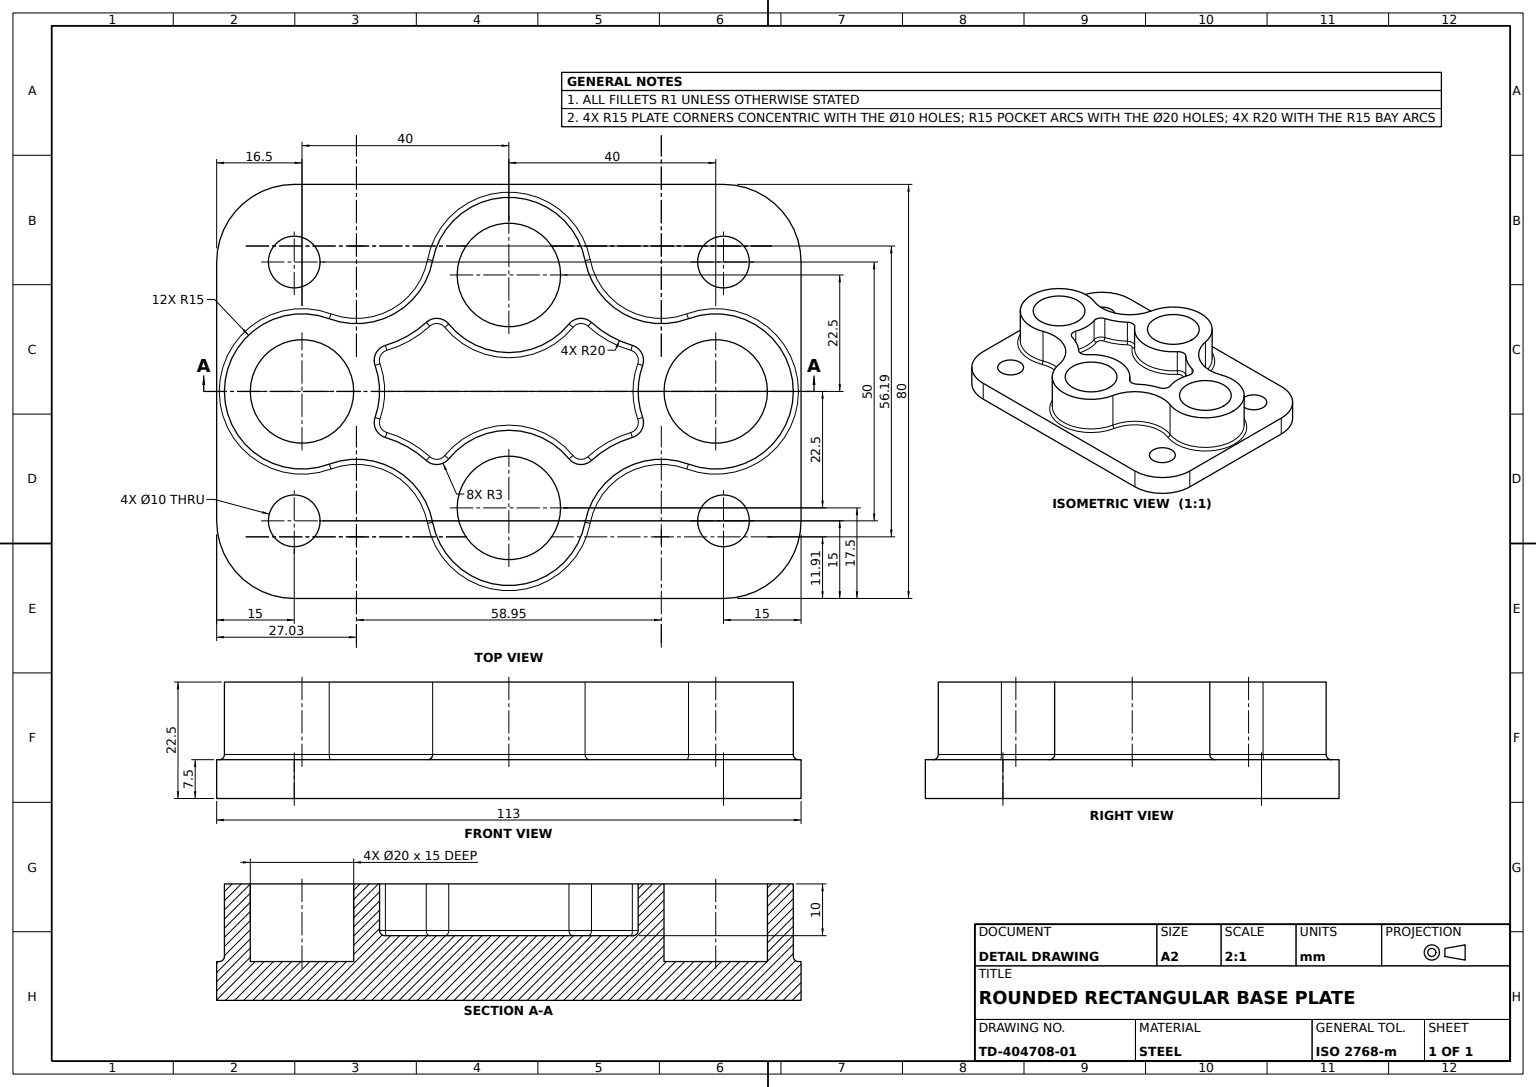
solid
v1 (0,22.5,-30)
v2 (0,7.5,-30)
e1 v1 v2 LINE
v3 (0,7.5,-50)
e2 v2 v3 CIRCLE(AX(P(0,7.5,-40),D(0,-1,0),D(0,0,1)),10)
v4 (0,22.5,-50)
e3 v4 v3 LINE
e4 v4 v1 CIRCLE(AX(P(0,22.5,-40),D(0,1,0),D(0,0,1)),10)
face CYL(AX(P(0,22.5,-40),D(0,-1,0),D(0,0,-1)),10) rev [e1 e2 -e3 e4]
v5 (5.01068,13.5,-25.861645)
v6 (8.892813,13.5,-23.873986)
e5 v5 v6 CIRCLE(AX(P(6.012816,13.5,-23.033974),D(0,-1,0),D(0,0,1)),3)
v7 (8.892813,22.5,-23.873986)
e6 v6 v7 LINE
v8 (5.01068,22.5,-25.861645)
e7 v7 v8 CIRCLE(AX(P(6.012816,22.5,-23.033974),D(0,1,0),D(0,0,-1)),3)
e8 v5 v8 LINE
face CYL(AX(P(6.012816,12.5,-23.033974),D(0,1,0),D(0,0,1)),3) rev [e5 e6 e7 -e8]
v9 (12.598841,12.5,-15.298823)
v10 (7.932814,12.5,-23.593982)
e9 v9 v10 CIRCLE(AX(P(28.092789,12.5,-29.474069),D(0,-1,0),D(0,0,1)),21)
v11 (13.336648,13.5,-15.973835)
e10 v9 v11 CIRCLE(AX(P(12.598841,13.5,-15.298823),D(0.675011674,0,0.737807048),D(0.737807048,0,-0.675011674)),1)
e11 v6 v11 CIRCLE(AX(P(28.092789,13.5,-29.474069),D(0,1,0),D(0,0,1)),20)
e12 v10 v6 CIRCLE(AX(P(7.932814,13.5,-23.593982),D(0.280004116,0,0.9599988),D(0.9599988,0,-0.280004116)),1)
face TORUS(AX(P(28.092789,13.5,-29.474069),D(0,1,0),D(0,0,1)),21,1) rev [-e9 e10 -e11 -e12]
v12 (0,7.5,50)
v13 (0,7.5,30)
e13 v12 v13 CIRCLE(AX(P(0,7.5,40),D(0,-1,0),D(0,0,1)),10)
e14 v13 v12 CIRCLE(AX(P(0,7.5,40),D(0,-1,0),D(0,0,1)),10)
face PLANE(AX(P(-25,7.5,41.5),D(0,1,0),D(0,0,1))) [-e13 -e14]
v14 (-8.892813,13.5,-23.873986)
v15 (-8.892813,22.5,-23.873986)
e15 v14 v15 LINE
v16 (-13.336648,22.5,-15.973835)
e16 v15 v16 CIRCLE(AX(P(-28.092789,22.5,-29.474069),D(0,-1,0),D(0,0,-1)),20)
v17 (-13.336648,13.5,-15.973835)
e17 v17 v16 LINE
e18 v17 v14 CIRCLE(AX(P(-28.092789,13.5,-29.474069),D(0,1,0),D(0,0,1)),20)
face CYL(AX(P(-28.092789,12.5,-29.474069),D(0,1,0),D(0,0,1)),20) [e15 e16 -e17 e18]
e19 v3 v2 CIRCLE(AX(P(0,7.5,-40),D(0,-1,0),D(0,0,1)),10)
face PLANE(AX(P(-25,7.5,41.5),D(0,1,0),D(0,0,1))) [-e2 -e19]
v18 (0,22.5,30)
e20 v18 v13 LINE
v19 (0,22.5,50)
e21 v18 v19 CIRCLE(AX(P(0,22.5,40),D(0,1,0),D(0,0,1)),10)
e22 v19 v12 LINE
face CYL(AX(P(0,22.5,40),D(0,-1,0),D(0,0,-1)),10) rev [-e20 e21 e22 e13]
v20 (-6.012816,12.5,25.033974)
v21 (-6.012816,13.5,26.033974)
e23 v20 v21 CIRCLE(AX(P(-6.012816,13.5,25.033974),D(-1,0,0),D(0,0,1)),1)
v22 (-5.01068,13.5,25.861645)
e24 v22 v21 CIRCLE(AX(P(-6.012816,13.5,23.033974),D(0,-1,0),D(0,0,1)),3)
v23 (-5.344724,12.5,24.919087)
e25 v22 v23 CIRCLE(AX(P(-5.344724,13.5,24.919087),D(0.942557427,0,-0.334044155),D(-0.334044155,0,-0.942557427)),1)
e26 v20 v23 CIRCLE(AX(P(-6.012816,12.5,23.033974),D(0,1,0),D(0,0,1)),2)
face TORUS(AX(P(-6.012816,13.5,23.033974),D(0,1,0),D(0,0,1)),2,1) rev [e23 -e24 e25 -e26]
v24 (5.01068,13.5,25.861645)
v25 (5.344724,12.5,24.919087)
e27 v24 v25 CIRCLE(AX(P(5.344724,13.5,24.919087),D(0.942557427,0,0.334044155),D(0.334044155,0,-0.942557427)),1)
v26 (6.012814,13.5,26.033973)
e28 v26 v24 CIRCLE(AX(P(6.012814,13.5,23.033969),D(0,-1,0),D(0,0,1)),3.000004)
v27 (6.012814,12.5,25.033973)
e29 v27 v26 CIRCLE(AX(P(6.012814,13.5,25.033973),D(-1,0,0),D(0,0,1)),1)
e30 v25 v27 CIRCLE(AX(P(6.012814,12.5,23.033969),D(0,1,0),D(0,0,1)),2.000004)
face TORUS(AX(P(6.012814,13.5,23.033969),D(0,1,0),D(0,0,1)),2.000004,1) rev [-e27 -e28 -e29 -e30]
v28 (25.296394,8.5,-14.737034)
v29 (14.046394,8.5,-34.737034)
e31 v28 v29 CIRCLE(AX(P(28.092789,8.5,-29.474069),D(0,-1,0),D(0,0,1)),15)
v30 (25.482821,7.5,-15.719503)
e32 v30 v28 CIRCLE(AX(P(25.482821,8.5,-15.719503),D(-0.982468951,0,-0.186426284),D(-0.186426284,0,0.982468951)),1)
v31 (14.982821,7.5,-34.38617)
e33 v31 v30 CIRCLE(AX(P(28.092789,7.5,-29.474069),D(0,1,0),D(0,0,1)),14)
e34 v31 v29 CIRCLE(AX(P(14.982821,8.5,-34.38617),D(0.350864382,0,-0.936426284),D(-0.936426284,0,-0.350864382)),1)
face TORUS(AX(P(28.092789,8.5,-29.474069),D(0,1,0),D(0,0,1)),14,1) rev [-e31 -e32 -e33 e34]
v32 (25,0,-36.5)
v33 (25,0,-46.5)
e35 v32 v33 CIRCLE(AX(P(25,0,-41.5),D(0,1,0),D(0,0,1)),5)
v34 (25,7.5,-36.5)
e36 v34 v32 LINE
v35 (25,7.5,-46.5)
e37 v34 v35 CIRCLE(AX(P(25,7.5,-41.5),D(0,1,0),D(0,0,1)),5)
e38 v35 v33 LINE
face CYL(AX(P(25,7.5,-41.5),D(0,-1,0),D(0,0,-1)),5) rev [-e35 -e36 e37 e38]
v36 (25,7.5,46.5)
v37 (25,0,46.5)
e39 v36 v37 LINE
v38 (25,7.5,36.5)
e40 v36 v38 CIRCLE(AX(P(25,7.5,41.5),D(0,1,0),D(0,0,1)),5)
v39 (25,0,36.5)
e41 v38 v39 LINE
e42 v37 v39 CIRCLE(AX(P(25,0,41.5),D(0,1,0),D(0,0,1)),5)
face CYL(AX(P(25,7.5,41.5),D(0,-1,0),D(0,0,-1)),5) rev [-e39 e40 e41 -e42]
v40 (-14.046394,8.5,34.737034)
v41 (0,8.5,55)
e43 v40 v41 CIRCLE(AX(P(0,8.5,40),D(0,1,0),D(0,0,1)),15)
v42 (-14.982821,7.5,34.38617)
e44 v40 v42 CIRCLE(AX(P(-14.982821,8.5,34.38617),D(0.350864382,0,-0.936426284),D(-0.936426284,0,-0.350864382)),1)
v43 (0,7.5,56)
e45 v43 v42 CIRCLE(AX(P(0,7.5,40),D(0,-1,0),D(0,0,1)),16)
e46 v41 v43 CIRCLE(AX(P(0,8.5,56),D(-1,0,0),D(0,0,1)),1)
face TORUS(AX(P(0,8.5,40),D(0,1,0),D(0,0,1)),16,1) rev [-e43 e44 -e45 -e46]
v44 (13.336648,13.5,15.973835)
v45 (13.336648,22.5,15.973835)
e47 v44 v45 LINE
v46 (8.892813,13.5,23.873986)
e48 v44 v46 CIRCLE(AX(P(28.092885,13.5,29.474123),D(0,1,0),D(0,0,1)),20.000108)
v47 (8.892813,22.5,23.873986)
e49 v46 v47 LINE
e50 v47 v45 CIRCLE(AX(P(28.092885,22.5,29.474123),D(0,-1,0),D(0,0,-1)),20.000108)
face CYL(AX(P(28.092885,12.5,29.474123),D(0,1,0),D(0,0,1)),20.000108) [-e47 e48 e49 e50]
v48 (22.5,7.5,-10)
v49 (22.5,7.5,10)
e51 v48 v49 CIRCLE(AX(P(22.5,7.5,0),D(0,-1,0),D(0,0,1)),10)
e52 v49 v48 CIRCLE(AX(P(22.5,7.5,0),D(0,-1,0),D(0,0,1)),10)
face PLANE(AX(P(-25,7.5,41.5),D(0,1,0),D(0,0,1))) [-e51 -e52]
v50 (-25.296394,22.5,-14.737034)
v51 (-25.296394,8.5,-14.737034)
e53 v50 v51 LINE
v52 (-25.296394,8.5,14.737034)
e54 v51 v52 CIRCLE(AX(P(-22.5,8.5,0),D(0,1,0),D(0,0,1)),15)
v53 (-25.296394,22.5,14.737034)
e55 v53 v52 LINE
e56 v50 v53 CIRCLE(AX(P(-22.5,22.5,0),D(0,1,0),D(0,0,1)),15)
face CYL(AX(P(-22.5,22.5,0),D(0,-1,0),D(0,0,-1)),15) [e53 e54 -e55 -e56]
e57 v39 v37 CIRCLE(AX(P(25,0,41.5),D(0,1,0),D(0,0,1)),5)
e58 v38 v36 CIRCLE(AX(P(25,7.5,41.5),D(0,1,0),D(0,0,1)),5)
face CYL(AX(P(25,7.5,41.5),D(0,-1,0),D(0,0,-1)),5) rev [e39 -e57 -e41 e58]
v54 (12.598841,12.5,15.298823)
e59 v44 v54 CIRCLE(AX(P(12.598841,13.5,15.298823),D(0.675011674,0,-0.737807048),D(-0.737807048,0,-0.675011674)),1)
v55 (7.932814,12.5,23.593981)
e60 v55 v54 CIRCLE(AX(P(28.092885,12.5,29.474123),D(0,-1,0),D(0,0,1)),21.000108)
e61 v46 v55 CIRCLE(AX(P(7.932814,13.5,23.593981),D(0.280005323,0,-0.959998447),D(-0.959998447,0,-0.280005323)),1)
face TORUS(AX(P(28.092885,13.5,29.474123),D(0,1,0),D(0,0,1)),21.000108,1) rev [-e48 e59 -e60 -e61]
v56 (-5.344725,12.5,-24.919088)
v57 (-7.932814,12.5,-23.593982)
e62 v56 v57 CIRCLE(AX(P(-6.012816,12.5,-23.033974),D(0,1,0),D(0,0,1)),2)
v58 (-5.01068,13.5,-25.861645)
e63 v56 v58 CIRCLE(AX(P(-5.344725,13.5,-24.919088),D(0.942557006,0,0.334045341),D(0.334045341,0,-0.942557006)),1)
e64 v14 v58 CIRCLE(AX(P(-6.012816,13.5,-23.033974),D(0,-1,0),D(0,0,1)),3)
e65 v57 v14 CIRCLE(AX(P(-7.932814,13.5,-23.593982),D(0.280004116,0,-0.9599988),D(-0.9599988,0,-0.280004116)),1)
face TORUS(AX(P(-6.012816,13.5,-23.033974),D(0,1,0),D(0,0,1)),2,1) rev [-e62 e63 -e64 -e65]
v59 (25,7.5,-56.5)
v60 (25,0,-56.5)
e66 v59 v60 LINE
v61 (-25,0,-56.5)
e67 v60 v61 LINE
v62 (-25,7.5,-56.5)
e68 v62 v61 LINE
e69 v59 v62 LINE
face PLANE(AX(P(-25,7.5,-56.5),D(0,0,1),D(1,0,0))) rev [e66 e67 -e68 -e69]
v63 (-12.598841,12.5,-15.298823)
e70 v63 v17 CIRCLE(AX(P(-12.598841,13.5,-15.298823),D(0.675011674,0,-0.737807048),D(-0.737807048,0,-0.675011674)),1)
e71 v57 v63 CIRCLE(AX(P(-28.092789,12.5,-29.474069),D(0,-1,0),D(0,0,1)),21)
face TORUS(AX(P(-28.092789,13.5,-29.474069),D(0,1,0),D(0,0,1)),21,1) rev [e65 -e18 -e70 -e71]
v64 (-13.019355,22.5,-11.624)
e72 v16 v64 CIRCLE(AX(P(-11.123226,22.5,-13.9488),D(0,1,0),D(0,0,1)),3)
v65 (-13.019355,13.5,-11.624)
e73 v65 v64 LINE
e74 v65 v17 CIRCLE(AX(P(-11.123226,13.5,-13.9488),D(0,-1,0),D(0,0,1)),3)
face CYL(AX(P(-11.123226,12.5,-13.9488),D(0,1,0),D(0,0,1)),3) rev [e17 e72 -e73 e74]
v66 (13.019355,22.5,11.624)
e75 v45 v66 CIRCLE(AX(P(11.123226,22.5,13.9488),D(0,1,0),D(0,0,1)),3)
v67 (13.019355,13.5,11.624)
e76 v67 v66 LINE
e77 v67 v44 CIRCLE(AX(P(11.123226,13.5,13.9488),D(0,-1,0),D(0,0,1)),3)
face CYL(AX(P(11.123226,12.5,13.9488),D(0,1,0),D(0,0,1)),3) rev [e47 e75 -e76 e77]
v68 (0,13.5,-25)
e78 v68 v5 CIRCLE(AX(P(0,13.5,-40),D(0,1,0),D(0,0,1)),15)
v69 (0,12.5,-24)
e79 v68 v69 CIRCLE(AX(P(0,13.5,-24),D(-1,0,0),D(0,0,1)),1)
v70 (5.344725,12.5,-24.919088)
e80 v70 v69 CIRCLE(AX(P(0,12.5,-40),D(0,-1,0),D(0,0,1)),16)
e81 v70 v5 CIRCLE(AX(P(5.344725,13.5,-24.919088),D(0.942557006,0,-0.334045341),D(-0.334045341,0,-0.942557006)),1)
face TORUS(AX(P(0,13.5,-40),D(0,1,0),D(0,0,1)),16,1) rev [-e78 e79 -e80 e81]
v71 (0,22.5,-25)
e82 v68 v71 LINE
v72 (-5.01068,22.5,-25.861645)
e83 v71 v72 CIRCLE(AX(P(0,22.5,-40),D(0,-1,0),D(0,0,1)),15)
e84 v58 v72 LINE
e85 v58 v68 CIRCLE(AX(P(0,13.5,-40),D(0,1,0),D(0,0,1)),15)
face CYL(AX(P(0,12.5,-40),D(0,1,0),D(0,0,1)),15) [e82 e83 -e84 e85]
e86 v33 v32 CIRCLE(AX(P(25,0,-41.5),D(0,1,0),D(0,0,1)),5)
v73 (-25,0,36.5)
v74 (-25,0,46.5)
e87 v73 v74 CIRCLE(AX(P(-25,0,41.5),D(0,1,0),D(0,0,1)),5)
e88 v74 v73 CIRCLE(AX(P(-25,0,41.5),D(0,1,0),D(0,0,1)),5)
v75 (-25,0,-46.5)
v76 (-25,0,-36.5)
e89 v75 v76 CIRCLE(AX(P(-25,0,-41.5),D(0,1,0),D(0,0,1)),5)
e90 v76 v75 CIRCLE(AX(P(-25,0,-41.5),D(0,1,0),D(0,0,1)),5)
v77 (-40,0,41.5)
v78 (-25,0,56.5)
e91 v77 v78 CIRCLE(AX(P(-25,0,41.5),D(0,1,0),D(0,0,1)),15)
v79 (-40,0,-41.5)
e92 v79 v77 LINE
e93 v61 v79 CIRCLE(AX(P(-25,0,-41.5),D(0,1,0),D(0,0,1)),15)
v80 (40,0,-41.5)
e94 v80 v60 CIRCLE(AX(P(25,0,-41.5),D(0,1,0),D(0,0,-1)),15)
v81 (40,0,41.5)
e95 v81 v80 LINE
v82 (25,0,56.5)
e96 v82 v81 CIRCLE(AX(P(25,0,41.5),D(0,1,0),D(0,0,1)),15)
e97 v78 v82 LINE
face PLANE(AX(P(-25,0,41.5),D(0,1,0),D(0,0,1))) rev [e42 e57] [e86 e35] [e87 e88] [e89 e90] [-e91 -e92 -e93 -e67 -e94 -e95 -e96 -e97]
v83 (22.5,22.5,-10)
e98 v83 v48 LINE
v84 (22.5,22.5,10)
e99 v83 v84 CIRCLE(AX(P(22.5,22.5,0),D(0,1,0),D(0,0,1)),10)
e100 v84 v49 LINE
face CYL(AX(P(22.5,22.5,0),D(0,-1,0),D(0,0,-1)),10) rev [e52 -e98 e99 e100]
e101 v24 v22 CIRCLE(AX(P(0,13.5,40.000056),D(0,1,0),D(0,0,1)),15.000053)
e102 v23 v25 CIRCLE(AX(P(0,12.5,40.000056),D(0,-1,0),D(0,0,1)),16.000053)
face TORUS(AX(P(0,13.5,40.000056),D(0,1,0),D(0,0,1)),16.000053,1) rev [-e101 e27 -e102 -e25]
v85 (-13.019355,22.5,11.624)
e103 v64 v85 CIRCLE(AX(P(-22.5,22.5,0),D(0,-1,0),D(0,0,-1)),15)
v86 (-13.019355,13.5,11.624)
e104 v86 v85 LINE
e105 v86 v65 CIRCLE(AX(P(-22.5,13.5,0),D(0,1,0),D(0,0,1)),15)
face CYL(AX(P(-22.5,12.5,0),D(0,1,0),D(0,0,1)),15) [e103 -e104 e105 e73]
v87 (-25.482821,7.5,-15.719503)
v88 (-14.982821,7.5,-34.38617)
e106 v87 v88 CIRCLE(AX(P(-28.092789,7.5,-29.474069),D(0,1,0),D(0,0,1)),14)
e107 v88 v31 CIRCLE(AX(P(0,7.5,-40),D(0,-1,0),D(0,0,1)),16)
v89 (25.482821,7.5,15.719503)
e108 v30 v89 CIRCLE(AX(P(22.5,7.5,0),D(0,-1,0),D(0,0,1)),16)
v90 (14.982821,7.5,34.38617)
e109 v89 v90 CIRCLE(AX(P(28.092789,7.5,29.474069),D(0,1,0),D(0,0,1)),14)
e110 v90 v43 CIRCLE(AX(P(0,7.5,40),D(0,-1,0),D(0,0,1)),16)
v91 (-25.482821,7.5,15.719503)
e111 v42 v91 CIRCLE(AX(P(-28.092789,7.5,29.474069),D(0,1,0),D(0,0,1)),14)
e112 v91 v87 CIRCLE(AX(P(-22.5,7.5,0),D(0,-1,0),D(0,0,1)),16)
e113 v35 v34 CIRCLE(AX(P(25,7.5,-41.5),D(0,1,0),D(0,0,1)),5)
v92 (-40,7.5,41.5)
v93 (-25,7.5,56.5)
e114 v92 v93 CIRCLE(AX(P(-25,7.5,41.5),D(0,1,0),D(0,0,1)),15)
v94 (25,7.5,56.5)
e115 v93 v94 LINE
v95 (40,7.5,41.5)
e116 v94 v95 CIRCLE(AX(P(25,7.5,41.5),D(0,1,0),D(0,0,1)),15)
v96 (40,7.5,-41.5)
e117 v95 v96 LINE
e118 v96 v59 CIRCLE(AX(P(25,7.5,-41.5),D(0,1,0),D(0,0,-1)),15)
v97 (-40,7.5,-41.5)
e119 v62 v97 CIRCLE(AX(P(-25,7.5,-41.5),D(0,1,0),D(0,0,1)),15)
e120 v97 v92 LINE
v98 (-25,7.5,36.5)
v99 (-25,7.5,46.5)
e121 v98 v99 CIRCLE(AX(P(-25,7.5,41.5),D(0,1,0),D(0,0,1)),5)
e122 v99 v98 CIRCLE(AX(P(-25,7.5,41.5),D(0,1,0),D(0,0,1)),5)
v100 (-25,7.5,-36.5)
v101 (-25,7.5,-46.5)
e123 v100 v101 CIRCLE(AX(P(-25,7.5,-41.5),D(0,1,0),D(0,0,1)),5)
e124 v101 v100 CIRCLE(AX(P(-25,7.5,-41.5),D(0,1,0),D(0,0,1)),5)
face PLANE(AX(P(-25,7.5,41.5),D(0,1,0),D(0,0,1))) [e106 e107 e33 e108 e109 e110 e45 e111 e112] [-e37 -e113] [e114 e115 e116 e117 e118 e69 e119 e120] [-e121 -e122] [-e123 -e124] [-e58 -e40]
e125 v72 v15 CIRCLE(AX(P(-6.012816,22.5,-23.033974),D(0,1,0),D(0,0,1)),3)
face CYL(AX(P(-6.012816,12.5,-23.033974),D(0,1,0),D(0,0,1)),3) rev [-e15 e64 e84 e125]
v102 (-12.387312,12.5,12.398933)
v103 (-12.598841,12.5,15.298823)
e126 v102 v103 CIRCLE(AX(P(-11.123226,12.5,13.9488),D(0,1,0),D(0,0,1)),2)
v104 (-7.932814,12.5,23.593982)
e127 v103 v104 CIRCLE(AX(P(-28.092789,12.5,29.474069),D(0,-1,0),D(0,0,1)),21)
e128 v104 v20 CIRCLE(AX(P(-6.012816,12.5,23.033974),D(0,1,0),D(0,0,1)),2)
e129 v27 v55 CIRCLE(AX(P(6.012814,12.5,23.033969),D(0,1,0),D(0,0,1)),2.000004)
v105 (12.387312,12.5,12.398933)
e130 v54 v105 CIRCLE(AX(P(11.123226,12.5,13.9488),D(0,1,0),D(0,0,1)),2)
v106 (12.387312,12.5,-12.398933)
e131 v105 v106 CIRCLE(AX(P(22.5,12.5,0),D(0,-1,0),D(0,0,1)),16)
e132 v106 v9 CIRCLE(AX(P(11.123226,12.5,-13.9488),D(0,1,0),D(0,0,1)),2)
e133 v10 v70 CIRCLE(AX(P(6.012816,12.5,-23.033974),D(0,1,0),D(0,0,1)),2)
e134 v69 v56 CIRCLE(AX(P(0,12.5,-40),D(0,-1,0),D(0,0,1)),16)
v107 (-12.387312,12.5,-12.398933)
e135 v63 v107 CIRCLE(AX(P(-11.123226,12.5,-13.9488),D(0,1,0),D(0,0,1)),2)
e136 v107 v102 CIRCLE(AX(P(-22.5,12.5,0),D(0,-1,0),D(0,0,1)),16)
face PLANE(AX(P(-17.052802,12.5,-26.254021),D(0,1,0),D(0,0,1))) [e126 e127 e128 e26 e102 e30 e129 e60 e130 e131 e132 e9 e133 e80 e134 e62 e71 e135 e136]
e137 v96 v80 LINE
e138 v95 v81 LINE
face PLANE(AX(P(40,7.5,-41.5),D(-1,0,0),D(0,0,1))) rev [-e137 -e117 e138 e95]
v108 (-14.046394,22.5,34.737034)
e139 v108 v40 LINE
e140 v53 v108 CIRCLE(AX(P(-28.092789,22.5,29.474069),D(0,-1,0),D(0,0,-1)),15)
e141 v52 v40 CIRCLE(AX(P(-28.092789,8.5,29.474069),D(0,-1,0),D(0,0,1)),15)
face CYL(AX(P(-28.092789,22.5,29.474069),D(0,-1,0),D(0,0,-1)),15) rev [-e139 -e140 e55 e141]
v109 (0,22.5,-55)
v110 (-14.046394,22.5,-34.737034)
e142 v109 v110 CIRCLE(AX(P(0,22.5,-40),D(0,1,0),D(0,0,1)),15)
v111 (0,8.5,-55)
e143 v109 v111 LINE
v112 (-14.046394,8.5,-34.737034)
e144 v111 v112 CIRCLE(AX(P(0,8.5,-40),D(0,1,0),D(0,0,1)),15)
e145 v110 v112 LINE
face CYL(AX(P(0,22.5,-40),D(0,-1,0),D(0,0,-1)),15) [-e142 e143 e144 -e145]
v113 (-22.5,22.5,10)
v114 (-22.5,7.5,10)
e146 v113 v114 LINE
v115 (-22.5,22.5,-10)
e147 v113 v115 CIRCLE(AX(P(-22.5,22.5,0),D(0,1,0),D(0,0,1)),10)
v116 (-22.5,7.5,-10)
e148 v115 v116 LINE
e149 v116 v114 CIRCLE(AX(P(-22.5,7.5,0),D(0,-1,0),D(0,0,1)),10)
face CYL(AX(P(-22.5,22.5,0),D(0,-1,0),D(0,0,-1)),10) rev [-e146 e147 e148 e149]
face TORUS(AX(P(0,13.5,-40),D(0,1,0),D(0,0,1)),16,1) rev [-e85 -e63 -e134 -e79]
v117 (14.046394,22.5,34.737034)
v118 (25.296394,22.5,14.737034)
e150 v117 v118 CIRCLE(AX(P(28.092789,22.5,29.474069),D(0,-1,0),D(0,0,1)),15)
v119 (14.046394,8.5,34.737034)
e151 v117 v119 LINE
v120 (25.296394,8.5,14.737034)
e152 v119 v120 CIRCLE(AX(P(28.092789,8.5,29.474069),D(0,-1,0),D(0,0,1)),15)
e153 v118 v120 LINE
face CYL(AX(P(28.092789,22.5,29.474069),D(0,-1,0),D(0,0,-1)),15) rev [-e150 e151 e152 -e153]
v121 (6.012814,22.5,26.033973)
e154 v26 v121 LINE
v122 (5.01068,22.5,25.861645)
e155 v24 v122 LINE
e156 v122 v121 CIRCLE(AX(P(6.012814,22.5,23.033969),D(0,1,0),D(0,0,1)),3.000004)
face CYL(AX(P(6.012814,12.5,23.033969),D(0,1,0),D(0,0,1)),3.000004) rev [-e154 e28 e155 e156]
e157 v41 v119 CIRCLE(AX(P(0,8.5,40),D(0,1,0),D(0,0,1)),15)
e158 v108 v117 CIRCLE(AX(P(0,22.5,40),D(0,1,0),D(0,0,1)),15)
face CYL(AX(P(0,22.5,40),D(0,-1,0),D(0,0,-1)),15) [e139 e43 e157 -e151 -e158]
e159 v89 v120 CIRCLE(AX(P(25.482821,8.5,15.719503),D(0.982468951,0,-0.186426284),D(-0.186426284,0,-0.982468951)),1)
e160 v90 v119 CIRCLE(AX(P(14.982821,8.5,34.38617),D(-0.350864382,0,-0.936426284),D(-0.936426284,0,0.350864382)),1)
face TORUS(AX(P(28.092789,8.5,29.474069),D(0,1,0),D(0,0,1)),14,1) rev [-e109 e159 -e152 -e160]
v123 (14.046394,22.5,-34.737034)
e161 v123 v29 LINE
v124 (25.296394,22.5,-14.737034)
e162 v124 v123 CIRCLE(AX(P(28.092789,22.5,-29.474069),D(0,-1,0),D(0,0,1)),15)
e163 v124 v28 LINE
face CYL(AX(P(28.092789,22.5,-29.474069),D(0,-1,0),D(0,0,-1)),15) rev [e31 -e161 -e162 e163]
e164 v52 v91 CIRCLE(AX(P(-25.482821,8.5,15.719503),D(-0.982468951,0,-0.186426284),D(-0.186426284,0,0.982468951)),1)
e165 v51 v87 CIRCLE(AX(P(-25.482821,8.5,-15.719503),D(0.982468951,0,-0.186426284),D(-0.186426284,0,-0.982468951)),1)
face TORUS(AX(P(-22.5,8.5,0),D(0,1,0),D(0,0,1)),16,1) rev [-e112 -e164 -e54 e165]
e166 v100 v76 LINE
e167 v101 v75 LINE
face CYL(AX(P(-25,7.5,-41.5),D(0,-1,0),D(0,0,-1)),5) rev [-e166 e123 e167 -e90]
face TORUS(AX(P(0,8.5,40),D(0,1,0),D(0,0,1)),16,1) rev [e46 -e110 e160 -e157]
e168 v105 v67 CIRCLE(AX(P(12.387312,13.5,12.398933),D(0.774933336,0,0.632042977),D(0.632042977,0,-0.774933336)),1)
v125 (13.019355,13.5,-11.624)
e169 v125 v67 CIRCLE(AX(P(22.5,13.5,0),D(0,1,0),D(0,0,1)),15)
e170 v106 v125 CIRCLE(AX(P(12.387312,13.5,-12.398933),D(-0.774933336,0,0.632042977),D(0.632042977,0,0.774933336)),1)
face TORUS(AX(P(22.5,13.5,0),D(0,1,0),D(0,0,1)),16,1) rev [-e131 e168 -e169 -e170]
e171 v114 v116 CIRCLE(AX(P(-22.5,7.5,0),D(0,-1,0),D(0,0,1)),10)
face PLANE(AX(P(-25,7.5,41.5),D(0,1,0),D(0,0,1))) [-e171 -e149]
e172 v98 v73 LINE
e173 v99 v74 LINE
face CYL(AX(P(-25,7.5,41.5),D(0,-1,0),D(0,0,-1)),5) rev [-e172 e121 e173 -e87]
e174 v65 v107 CIRCLE(AX(P(-12.387312,13.5,-12.398933),D(0.774933336,0,0.632042977),D(0.632042977,0,-0.774933336)),1)
face TORUS(AX(P(-11.123226,13.5,-13.9488),D(0,1,0),D(0,0,1)),2,1) rev [e70 -e74 e174 -e135]
e175 v29 v111 CIRCLE(AX(P(0,8.5,-40),D(0,1,0),D(0,0,1)),15)
e176 v123 v109 CIRCLE(AX(P(0,22.5,-40),D(0,1,0),D(0,0,1)),15)
face CYL(AX(P(0,22.5,-40),D(0,-1,0),D(0,0,-1)),15) [e175 -e143 -e176 e161]
face CYL(AX(P(25,7.5,-41.5),D(0,-1,0),D(0,0,-1)),5) rev [-e38 e113 e36 -e86]
e177 v94 v82 LINE
face CYL(AX(P(25,7.5,41.5),D(0,-1,0),D(0,0,-1)),15) [e96 -e138 -e116 e177]
v126 (13.336648,22.5,-15.973835)
e178 v11 v126 LINE
e179 v11 v125 CIRCLE(AX(P(11.123226,13.5,-13.9488),D(0,-1,0),D(0,0,1)),3)
v127 (13.019355,22.5,-11.624)
e180 v125 v127 LINE
e181 v127 v126 CIRCLE(AX(P(11.123226,22.5,-13.9488),D(0,1,0),D(0,0,-1)),3)
face CYL(AX(P(11.123226,12.5,-13.9488),D(0,1,0),D(0,0,1)),3) rev [-e178 e179 e180 e181]
e182 v112 v88 CIRCLE(AX(P(-14.982821,8.5,-34.38617),D(-0.350864382,0,-0.936426284),D(-0.936426284,0,0.350864382)),1)
face TORUS(AX(P(0,8.5,-40),D(0,1,0),D(0,0,1)),16,1) rev [-e175 -e34 -e107 -e182 -e144]
v128 (-5.01068,22.5,25.861645)
e183 v22 v128 LINE
e184 v128 v122 CIRCLE(AX(P(0,22.5,40.000056),D(0,-1,0),D(0,0,-1)),15.000053)
face CYL(AX(P(0,12.5,40.000056),D(0,1,0),D(0,0,1)),15.000053) [-e155 e101 e183 e184]
e185 v118 v124 CIRCLE(AX(P(22.5,22.5,0),D(0,1,0),D(0,0,1)),15)
e186 v110 v50 CIRCLE(AX(P(-28.092789,22.5,-29.474069),D(0,-1,0),D(0,0,-1)),15)
e187 v84 v83 CIRCLE(AX(P(22.5,22.5,0),D(0,1,0),D(0,0,1)),10)
e188 v1 v4 CIRCLE(AX(P(0,22.5,-40),D(0,1,0),D(0,0,1)),10)
e189 v19 v18 CIRCLE(AX(P(0,22.5,40),D(0,1,0),D(0,0,1)),10)
e190 v66 v127 CIRCLE(AX(P(22.5,22.5,0),D(0,-1,0),D(0,0,1)),15)
e191 v121 v47 CIRCLE(AX(P(6.012814,22.5,23.033969),D(0,1,0),D(0,0,1)),3.000004)
v129 (-6.012816,22.5,26.033974)
e192 v129 v128 CIRCLE(AX(P(-6.012816,22.5,23.033974),D(0,1,0),D(0,0,1)),3)
v130 (-8.892813,22.5,23.873986)
e193 v130 v129 CIRCLE(AX(P(-6.012816,22.5,23.033974),D(0,1,0),D(0,0,1)),3)
v131 (-13.336648,22.5,15.973835)
e194 v131 v130 CIRCLE(AX(P(-28.092789,22.5,29.474069),D(0,-1,0),D(0,0,-1)),20)
e195 v85 v131 CIRCLE(AX(P(-11.123226,22.5,13.9488),D(0,1,0),D(0,0,1)),3)
e196 v8 v71 CIRCLE(AX(P(0,22.5,-40),D(0,-1,0),D(0,0,1)),15)
e197 v126 v7 CIRCLE(AX(P(28.092789,22.5,-29.474069),D(0,-1,0),D(0,0,1)),20)
e198 v115 v113 CIRCLE(AX(P(-22.5,22.5,0),D(0,1,0),D(0,0,1)),10)
face PLANE(AX(P(-14.046394,22.5,-34.737034),D(0,1,0),D(0,0,1))) [e150 e185 e162 e176 e142 e186 e56 e140 e158] [-e187 -e99] [-e4 -e188] [-e189 -e21] [-e181 -e190 -e75 -e50 -e191 -e156 -e184 -e192 -e193 -e194 -e195 -e103 -e72 -e16 -e125 -e83 -e196 -e7 -e197] [-e198 -e147]
v132 (-8.892813,13.5,23.873986)
e199 v132 v104 CIRCLE(AX(P(-7.932814,13.5,23.593982),D(0.280004116,0,0.9599988),D(0.9599988,0,-0.280004116)),1)
e200 v21 v132 CIRCLE(AX(P(-6.012816,13.5,23.033974),D(0,-1,0),D(0,0,1)),3)
face TORUS(AX(P(-6.012816,13.5,23.033974),D(0,1,0),D(0,0,1)),2,1) rev [-e199 -e200 -e23 -e128]
e201 v92 v77 LINE
e202 v97 v79 LINE
face PLANE(AX(P(-40,7.5,-41.5),D(1,0,0),D(0,0,-1))) rev [e92 -e201 -e120 e202]
face TORUS(AX(P(-28.092789,8.5,29.474069),D(0,1,0),D(0,0,1)),14,1) rev [-e141 e164 -e111 -e44]
face CYL(AX(P(0,22.5,40),D(0,-1,0),D(0,0,-1)),10) rev [e189 e20 e14 -e22]
face TORUS(AX(P(11.123226,13.5,13.9488),D(0,1,0),D(0,0,1)),2,1) rev [-e77 -e168 -e130 -e59]
e203 v93 v78 LINE
face PLANE(AX(P(-25,7.5,56.5),D(0,0,-1),D(-1,0,0))) rev [e203 e97 -e177 -e115]
v133 (-13.336648,13.5,15.973835)
e204 v133 v131 LINE
e205 v133 v86 CIRCLE(AX(P(-11.123226,13.5,13.9488),D(0,-1,0),D(0,0,1)),3)
face CYL(AX(P(-11.123226,12.5,13.9488),D(0,1,0),D(0,0,1)),3) rev [e104 e195 -e204 e205]
face CYL(AX(P(25,7.5,-41.5),D(0,-1,0),D(0,0,-1)),15) [e94 -e66 -e118 e137]
e206 v112 v51 CIRCLE(AX(P(-28.092789,8.5,-29.474069),D(0,-1,0),D(0,0,1)),15)
face CYL(AX(P(-28.092789,22.5,-29.474069),D(0,-1,0),D(0,0,-1)),15) rev [-e186 e145 e206 -e53]
face CYL(AX(P(22.5,22.5,0),D(0,-1,0),D(0,0,-1)),10) rev [e187 e98 e51 -e100]
e207 v46 v26 CIRCLE(AX(P(6.012814,13.5,23.033969),D(0,-1,0),D(0,0,1)),3.000004)
face CYL(AX(P(6.012814,12.5,23.033969),D(0,1,0),D(0,0,1)),3.000004) rev [-e49 e207 e154 e191]
face CYL(AX(P(0,22.5,-40),D(0,-1,0),D(0,0,-1)),10) rev [e19 -e1 e188 e3]
face TORUS(AX(P(11.123226,13.5,-13.9488),D(0,1,0),D(0,0,1)),2,1) rev [-e179 -e10 -e132 e170]
face CYL(AX(P(-25,7.5,-41.5),D(0,-1,0),D(0,0,-1)),15) [-e119 e68 e93 -e202]
e208 v120 v28 CIRCLE(AX(P(22.5,8.5,0),D(0,1,0),D(0,0,1)),15)
face TORUS(AX(P(22.5,8.5,0),D(0,1,0),D(0,0,1)),16,1) rev [-e108 e32 -e208 -e159]
e209 v132 v130 LINE
e210 v132 v133 CIRCLE(AX(P(-28.092789,13.5,29.474069),D(0,1,0),D(0,0,1)),20)
face CYL(AX(P(-28.092789,12.5,29.474069),D(0,1,0),D(0,0,1)),20) [e204 e194 -e209 e210]
face CYL(AX(P(22.5,12.5,0),D(0,1,0),D(0,0,1)),15) [e76 e190 -e180 e169]
face CYL(AX(P(-22.5,22.5,0),D(0,-1,0),D(0,0,-1)),10) rev [-e148 e198 e146 e171]
face CYL(AX(P(28.092789,12.5,-29.474069),D(0,1,0),D(0,0,1)),20) [e11 e178 e197 -e6]
face CYL(AX(P(0,12.5,-40),D(0,1,0),D(0,0,1)),15) [e196 -e82 e78 e8]
e211 v21 v129 LINE
face CYL(AX(P(-6.012816,12.5,23.033974),D(0,1,0),D(0,0,1)),3) rev [-e211 e200 e209 e193]
face CYL(AX(P(-25,7.5,41.5),D(0,-1,0),D(0,0,-1)),15) [-e114 e201 e91 -e203]
e212 v86 v102 CIRCLE(AX(P(-12.387312,13.5,12.398933),D(-0.774933336,0,0.632042977),D(0.632042977,0,0.774933336)),1)
face TORUS(AX(P(-22.5,13.5,0),D(0,1,0),D(0,0,1)),16,1) rev [-e136 -e174 -e105 e212]
face CYL(AX(P(22.5,22.5,0),D(0,-1,0),D(0,0,-1)),15) [-e163 -e185 e153 e208]
e213 v133 v103 CIRCLE(AX(P(-12.598841,13.5,15.298823),D(0.675011674,0,0.737807048),D(0.737807048,0,-0.675011674)),1)
face TORUS(AX(P(-28.092789,13.5,29.474069),D(0,1,0),D(0,0,1)),21,1) rev [e199 -e127 -e213 -e210]
face CYL(AX(P(-6.012816,12.5,23.033974),D(0,1,0),D(0,0,1)),3) rev [e24 e211 e192 -e183]
face CYL(AX(P(-25,7.5,41.5),D(0,-1,0),D(0,0,-1)),5) rev [e172 -e88 -e173 e122]
face TORUS(AX(P(-11.123226,13.5,13.9488),D(0,1,0),D(0,0,1)),2,1) rev [-e205 e213 -e126 -e212]
face TORUS(AX(P(-28.092789,8.5,-29.474069),D(0,1,0),D(0,0,1)),14,1) rev [-e206 e182 -e106 -e165]
face TORUS(AX(P(6.012814,13.5,23.033969),D(0,1,0),D(0,0,1)),2.000004,1) rev [-e207 e61 -e129 e29]
face CYL(AX(P(-25,7.5,-41.5),D(0,-1,0),D(0,0,-1)),5) rev [e124 e166 -e89 -e167]
face TORUS(AX(P(6.012816,13.5,-23.033974),D(0,1,0),D(0,0,1)),2,1) rev [-e81 -e133 e12 -e5]
